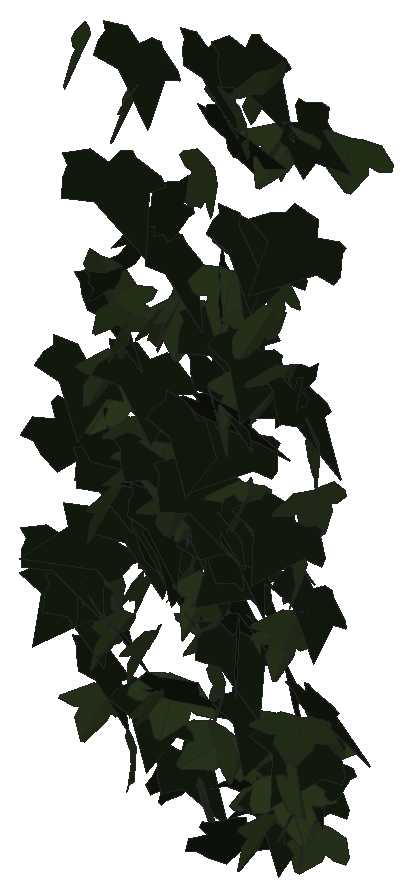
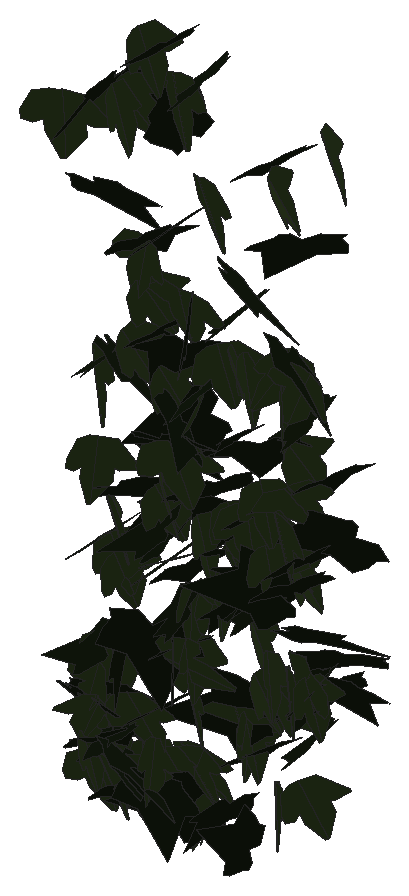
# SketchUp Ruby script. Lengths in inches.
U = 1.inch
M = Sketchup.active_model
def pt(a) = Geom::Point3d.new(a.map { |v| v * U })
def face(e, loops, mat)
  f = e.add_face(loops[0].map { |a| pt(a) })
  loops[1..].each { |l| e.add_face(l.map { |a| pt(a) }).erase! }
  f.material = f.back_material = mat if mat
  f
end
# faces: each face lists its corners as indices into pts; further lists are holes
def faces(e, pts, list, mat = nil) = list.each { |f| face(e, (f[0].is_a?(Array) ? f : [f]).map { |l| l.map { |i| pts[i] } }, mat) }
# xy, xz, yz: faces in a plane at the given z, y or x. An outline is a flat list of corners, or four numbers for a rectangle; further outlines are holes
def ring(l) = l.size == 4 ? [[l[0], l[1]], [l[2], l[1]], [l[2], l[3]], [l[0], l[3]]] : l.each_slice(2).to_a
def flat(e, list, mat, &to3) = list.each { |f| face(e, (f[0].is_a?(Array) ? f : [f]).map { |l| ring(l).map { |u, v| to3.(u, v) } }, mat) }
def xy(e, z, list, mat = nil) = flat(e, list, mat) { |x, y| [x, y, z] }
def xz(e, y, list, mat = nil) = flat(e, list, mat) { |x, z| [x, y, z] }
def yz(e, x, list, mat = nil) = flat(e, list, mat) { |y, z| [x, y, z] }
def lines(e, pts, list) = list.each { |a, b| e.add_line(pt(pts[a]), pt(pts[b])) }
# prism: a flat outline (further loops are holes) pulled along v
def prism(e, loops, v, mat = nil)
  f = face(e, loops, mat); d = Geom::Vector3d.new(v.map { |x| x * U })
  f.pushpull(f.normal.samedirection?(d) ? d.length : -d.length)
end
def box(e, o, s, mat = nil) = prism(e, [[o, [o[0] + s[0], o[1], o[2]], [o[0] + s[0], o[1] + s[1], o[2]], [o[0], o[1] + s[1], o[2]]]], [0, 0, s[2]], mat)
def at(x, y, z, deg = 0) = Geom::Transformation.translation(pt([x, y, z])) * Geom::Transformation.rotation(ORIGIN, Z_AXIS, deg.degrees)
def axes(o, x, y, z) = Geom::Transformation.new([*x, 0, *y, 0, *z, 0, *pt(o).to_a, 1])
def part(name) = M.definitions.add(name)
# library, detail: a bought-in or finely detailed component or shape, given as its bounding box
def library(name, o, s) = part(name).tap { |d| box(d.entities, o, s) }
def detail(e, o, s) = box(e.add_group.entities, o, s)
def put(e, d, t, mat = nil) = e.add_instance(d, t).tap { |i| i.material = mat if mat }
def group(e, t, mat = nil) = e.add_group.tap { |g| g.transformation = t; g.material = mat if mat }.entities
root = M.entities
M.materials.add("1026 AP 7946 SUNNY SIDE UP").color = [254, 231, 186]
M.materials.add("efeu1").color = [18, 25, 13]
M.materials.add("efeu2").color = [43, 57, 29]
c1 = part("ivyleaf_9")
p = [[1.54,2.16,1.25],[1.36,2.04,1.19],[-0.21,0.99,0.68],[-0.71,1.11,0.82],[-0.85,0.86,0.67],[-0.8,0.17,0.21],
  [-0.9,-0.01,0.1],[-0.67,-0.16,-0.02],[-0.08,-0.08,-0.05],[-0.03,-0.6,-0.4],[0.65,-0.88,-0.66],[0.83,-0.6,-0.49],
  [1.29,-0.42,-0.43],[1.8125,-0.07,-0.26],[1.21,0.44,0.15]]
faces(c1.entities,p,[[0,1,2,3,4,5,6,7,8,9,10,11,12,13,14]],"efeu1")
c2 = part("ivyleaf_10")
p = [[0,0.5,-0.03],[-0.0625,2.02,-0.43],[-0.19,2.01,-0.46],[-0.54,1.05,-0.29],[-0.52,0.625,-0.18],[-0.83,0.76,-0.28],
  [-1.16,0.64,-0.33],[-1.15,0.33,-0.24],[-0.77,-0.39,0.02],[-0.3,-0.51,0.16],[0.04,-0.48,0.23],[-0.02,2.01,-0.4375],
  [-0.06,2.01,-0.43],[0.04,-0.49,0.23],[0.67,-0.49,0.14],[1.38,0.36,-0.2],[1.375,0.51,-0.24],[0.81,0.65,-0.19],
  [0.62,0.59,-0.15],[0.6,1.09,-0.28],[0.5,1.23,-0.31]]
faces(c2.entities,p,[[0,1,2,3,4,5,6,7,8,9,10],[11,12,0,13,14,15,16,17,18,19,20]],"efeu2")
put(root,c1,axes([121.98,212.34,282.11],[-0.4716,-0.12043,-0.03746],[0.06512,-0.00764,-0.3322],[0.18645,-0.30194,0.02129]),"1026 AP 7946 SUNNY SIDE UP")
put(root,c2,axes([122.47,212.32,283.62],[0.07982,-0.31005,0.11549],[0.01592,-0.11369,-0.32422],[0.51911,0.05116,-0.00781]),"1026 AP 7946 SUNNY SIDE UP")
put(root,c1,axes([124.34,212.375,289.46],[0.07337,-0.12102,0.34642],[0.30772,-0.27593,-0.13163],[0.47142,0.19895,0.03201]),"1026 AP 7946 SUNNY SIDE UP")
put(root,c2,axes([125.5,212.28,282.88],[-0.20224,-0.29102,0.07419],[-0.01458,-0.07625,-0.32746],[0.47181,-0.1271,0.02168]),"1026 AP 7946 SUNNY SIDE UP")
put(root,c2,axes([125.39,212.33,282.65],[-0.14641,-0.29461,0.11515],[0.04803,-0.12613,-0.31235],[0.49408,-0.07504,0.06448]),"1026 AP 7946 SUNNY SIDE UP")
put(root,c2,axes([123.88,212.42,282.69],[-0.06359,-0.22295,0.24256],[0.12672,-0.23798,-0.2181],[0.49536,0.03226,0.08693]),"1026 AP 7946 SUNNY SIDE UP")
put(root,c2,axes([125.38,212.2,280.39],[0.3979,0.18623,0.0915],[0.1379,0.0283,-0.32221],[-0.29287,0.26634,-0.02741]),"1026 AP 7946 SUNNY SIDE UP")
put(root,c1,axes([122.46,212.29,288.4375],[-0.09486,-0.31906,-0.17967],[0.11042,0.16139,-0.33169],[0.55961,-0.08593,0.03499]),"1026 AP 7946 SUNNY SIDE UP")
put(root,c1,axes([124.34,212.03,279.43],[0.08612,0.14579,-0.28237],[0.14093,0.25993,0.16191],[0.46857,-0.10497,0.0032]),"1026 AP 7946 SUNNY SIDE UP")
put(root,c2,axes([125.61,212.26,281.38],[-0.3918,-0.209,0.04614],[-0.03482,-0.045,-0.33466],[0.33468,-0.24935,0.01919]),"1026 AP 7946 SUNNY SIDE UP")
put(root,c1,axes([123.72,212.48,285.05],[-0.12021,-0.32303,0.09626],[-0.00443,-0.09708,-0.34199],[0.52955,-0.07414,0.01899]),"1026 AP 7946 SUNNY SIDE UP")
put(root,c2,axes([124.93,212.41,279.61],[0.00787,-0.27161,0.17281],[0.01371,-0.16913,-0.2808],[0.50306,0.00886,0.00495]),"1026 AP 7946 SUNNY SIDE UP")
put(root,c2,axes([122.54,212.43,281.72],[0.00962,-0.26489,0.19993],[0.01872,-0.19531,-0.27404],[0.51741,0.01199,0.0062]),"1026 AP 7946 SUNNY SIDE UP")
put(root,c1,axes([123.28,212.51,282.92],[0.00139,-0.22449,0.25658],[0.02304,-0.25007,-0.23254],[0.52821,0.0115,0.00947]),"1026 AP 7946 SUNNY SIDE UP")
put(root,c1,axes([123.11,212.47,280.73],[-0.15088,-0.29808,0.07784],[0.0184,-0.08438,-0.32097],[0.48384,-0.08974,0.03648]),"1026 AP 7946 SUNNY SIDE UP")
put(root,c1,axes([122.2,212.38,281.18],[0.14885,-0.30447,0.0188],[-0.0019,-0.0213,-0.32851],[0.47977,0.09438,-0.00714]),"1026 AP 7946 SUNNY SIDE UP")
put(root,c2,axes([122.9,212.19,280.05],[0.20398,-0.25965,-0.14636],[0.00861,0.15566,-0.29003],[0.46421,0.11121,0.06969]),"1026 AP 7946 SUNNY SIDE UP")
put(root,c2,axes([123.58,212.3,283.99],[-0.16181,-0.31981,0.00986],[-0.00055,-0.01185,-0.34616],[0.5032,-0.10285,0.00279]),"1026 AP 7946 SUNNY SIDE UP")
put(root,c1,axes([124.7,212.51,286.4],[-0.13871,-0.31108,0.10614],[-0.01949,-0.10528,-0.33332],[0.51579,-0.08763,0.01595]),"1026 AP 7946 SUNNY SIDE UP")
put(root,c1,axes([121.9375,212.35,282.08],[-0.0157,-0.30585,-0.11025],[-0.00953,0.10549,-0.3145],[0.50853,-0.00747,-0.0093]),"1026 AP 7946 SUNNY SIDE UP")
put(root,c1,axes([123.85,212.34,284.39],[0.043,-0.35183,-0.15438],[0.05737,0.14997,-0.3598],[0.59734,0.01092,0.04567]),"1026 AP 7946 SUNNY SIDE UP")
put(root,c2,axes([123.45,212.33,281.13],[0.4817,0.10245,-0.03466],[-0.03828,-0.03479,-0.33198],[-0.16548,0.30629,-0.0241]),"1026 AP 7946 SUNNY SIDE UP")
put(root,c2,axes([123.03,212.37,281.71],[0.02886,-0.31487,0.06319],[-0.00167,-0.06329,-0.32526],[0.50495,0.01779,-0.00469]),"1026 AP 7946 SUNNY SIDE UP")
put(root,c1,axes([123.11,212.48,283.58],[0.06851,-0.32896,0.07609],[0.00669,-0.07582,-0.34225],[0.53074,0.04342,-0.00551]),"1026 AP 7946 SUNNY SIDE UP")
put(root,c1,axes([121.66,212.39,282.65],[-0.10323,-0.28278,-0.15401],[0.23333,0.10662,-0.27726],[0.44423,-0.12171,0.10984]),"1026 AP 7946 SUNNY SIDE UP")
put(root,c1,axes([124.45,212.57,283.15],[-0.31501,-0.19963,0.17381],[-0.04205,-0.1971,-0.2723],[0.40999,-0.1736,0.10562]),"1026 AP 7946 SUNNY SIDE UP")
put(root,c2,axes([125.3125,212.46,289.74],[-0.28616,-0.237,0.19736],[-0.06715,-0.20262,-0.29911],[0.4758,-0.17113,0.07648]),"1026 AP 7946 SUNNY SIDE UP")
put(root,c1,axes([123.33,212.2,281.125],[0.40036,-0.00071,0.20678],[0.31555,0.00781,-0.26217],[-0.00673,0.32413,0.00866]),"1026 AP 7946 SUNNY SIDE UP")
put(root,c2,axes([121.95,212.35,290.03],[0.21551,-0.3307,-0.02537],[-0.01643,0.02029,-0.36866],[0.52096,0.13744,-0.00113]),"1026 AP 7946 SUNNY SIDE UP")
put(root,c1,axes([124.46,212.53,283.46],[0.10075,-0.28666,0.17582],[0.04375,-0.17025,-0.30347],[0.52407,0.06932,-0.00847]),"1026 AP 7946 SUNNY SIDE UP")
put(root,c2,axes([125.64,212.14,280.33],[-0.04654,0.27766,-0.20714],[-0.0628,0.19924,0.28841],[0.53684,0.04738,0.01578]),"1026 AP 7946 SUNNY SIDE UP")
put(root,c2,axes([123.24,212.35,280.96],[-0.02999,-0.31993,-0.01573],[0.01456,0.01292,-0.32998],[0.50329,-0.01944,0.00861]),"1026 AP 7946 SUNNY SIDE UP")
put(root,c1,axes([121.87,212.54,285.23],[-0.13038,-0.32634,0.05369],[-0.00101,-0.05548,-0.34695],[0.52011,-0.08192,0.01279]),"1026 AP 7946 SUNNY SIDE UP")
put(root,c1,axes([123.03,212.47,282.96],[0.24152,-0.28204,0.07856],[0.03383,-0.07681,-0.33082],[0.45882,0.15413,-0.01696]),"1026 AP 7946 SUNNY SIDE UP")
put(root,c2,axes([124.9375,212.4,290.56],[-0.0761,-0.35302,0.02445],[0.0011,-0.02608,-0.36721],[0.55657,-0.04822,0.00407]),"1026 AP 7946 SUNNY SIDE UP")
put(root,c1,axes([124.31,212.3,283.96],[0.04677,-0.22517,-0.25324],[0.1103,0.24424,-0.22147],[0.51093,-0.03211,0.07099]),"1026 AP 7946 SUNNY SIDE UP")
put(root,c1,axes([122.97,212.48,283.41],[-0.25344,-0.25116,-0.14727],[0.24254,0.06186,-0.29369],[0.38297,-0.20538,0.08854]),"1026 AP 7946 SUNNY SIDE UP")
put(root,c2,axes([124.81,212.5,286.96],[-0.1432,-0.28736,0.16861],[-0.01065,-0.16978,-0.30889],[0.52116,-0.08242,0.04002]),"1026 AP 7946 SUNNY SIDE UP")
put(root,c2,axes([125.47,212.3,280.1],[0.10436,-0.29396,-0.11603],[-0.00971,0.11216,-0.30927],[0.49395,0.06431,0.01844]),"1026 AP 7946 SUNNY SIDE UP")
put(root,c1,axes([122.35,212.52,282.8],[-0.46019,-0.02794,0.14917],[-0.20323,-0.10704,-0.2907],[0.11217,-0.30856,0.08531]),"1026 AP 7946 SUNNY SIDE UP")
put(root,c2,axes([122.3,212.53,285.41],[-0.05315,-0.2918,0.17885],[0.02478,-0.17728,-0.30197],[0.53466,-0.0208,0.03177]),"1026 AP 7946 SUNNY SIDE UP")
put(root,c2,axes([124.49,212.26,289.96],[0.39965,-0.1725,-0.1954],[-0.10129,0.21428,-0.28995],[0.38903,0.23301,0.12524]),"1026 AP 7946 SUNNY SIDE UP")
put(root,c1,axes([125.18,212.62,284.02],[-0.30683,-0.25694,0.08238],[-0.02483,-0.08945,-0.33031],[0.42309,-0.19159,0.04036]),"1026 AP 7946 SUNNY SIDE UP")
put(root,c2,axes([123.28,212.3125,281.01],[-0.01538,-0.29711,-0.15278],[0.02307,0.14614,-0.30525],[0.52045,-0.01526,0.00901]),"1026 AP 7946 SUNNY SIDE UP")
put(root,c2,axes([122.68,212.26,286.51],[-0.20494,-0.22646,-0.23116],[0.20839,0.18046,-0.26741],[0.45434,-0.18492,0.01838]),"1026 AP 7946 SUNNY SIDE UP")
put(root,c1,axes([124.45,212.64,288],[-0.0305,-0.33944,0.09793],[-0.00525,-0.09695,-0.35082],[0.55508,-0.01957,0.00206]),"1026 AP 7946 SUNNY SIDE UP")
put(root,c1,axes([122.08,212.49,281.94],[0.33523,-0.2461,0.01976],[-0.00104,-0.02775,-0.33505],[0.38832,0.21238,-0.01795]),"1026 AP 7946 SUNNY SIDE UP")
put(root,c2,axes([122.2,212.53,280.49],[-0.22903,-0.26725,0.12402],[-0.02738,-0.12797,-0.31121],[0.46107,-0.14036,0.04312]),"1026 AP 7946 SUNNY SIDE UP")
put(root,c1,axes([121.6,212.34,284.39],[0.131,-0.10674,-0.32984],[0.3227,0.27715,-0.03863],[0.42016,-0.17959,0.13251]),"1026 AP 7946 SUNNY SIDE UP")
put(root,c1,axes([125.53,212.58,280.92],[-0.42097,-0.16263,-0.03561],[0.0694,-0.00816,-0.3213],[0.25174,-0.26971,0.02904]),"1026 AP 7946 SUNNY SIDE UP")
put(root,c2,axes([125.02,212.5625,286.16],[-0.0173,-0.32197,0.13866],[-0.01208,-0.13624,-0.33267],[0.54971,-0.01313,-0.00295]),"1026 AP 7946 SUNNY SIDE UP")
put(root,c2,axes([125.46,212.4,283.53],[0.22409,-0.28692,-0.11677],[-0.07305,0.10166,-0.32942],[0.4786,0.14985,0.0044]),"1026 AP 7946 SUNNY SIDE UP")
put(root,c1,axes([125.49,212.65,283.14],[-0.04575,-0.31576,0.10912],[0.01345,-0.1088,-0.32681],[0.52442,-0.02476,0.0179]),"1026 AP 7946 SUNNY SIDE UP")
put(root,c2,axes([124.42,212.59,285.85],[-0.08887,-0.29048,0.16641],[0.05685,-0.16988,-0.29963],[0.52079,-0.03102,0.0611]),"1026 AP 7946 SUNNY SIDE UP")
put(root,c1,axes([125.55,212.6,288.32],[-0.52722,-0.08548,-0.01484],[0.03195,-0.02355,-0.35545],[0.13238,-0.33476,0.0267]),"1026 AP 7946 SUNNY SIDE UP")
put(root,c2,axes([124.07,212.4375,285.53],[-0.17064,0.31483,-0.05166],[0.01132,-0.05243,-0.34321],[-0.5016,-0.10829,0.00983]),"1026 AP 7946 SUNNY SIDE UP")
put(root,c2,axes([124.54,212.46,284.23],[0.13973,-0.32884,-0.05482],[-0.01609,0.05042,-0.35061],[0.52309,0.08939,0.00386]),"1026 AP 7946 SUNNY SIDE UP")
put(root,c2,axes([123.6875,212.36,282.96],[0.02475,-0.27978,-0.17698],[-0.01887,0.16979,-0.28768],[0.51459,0.01968,-0.00204]),"1026 AP 7946 SUNNY SIDE UP")
put(root,c1,axes([123.82,212.62,290.45],[0.13275,-0.34153,0.05339],[0.00534,-0.05452,-0.36261],[0.54361,0.08394,-0.00948]),"1026 AP 7946 SUNNY SIDE UP")
put(root,c2,axes([125.78,212.3,285.5],[0.28543,-0.23687,-0.25889],[-0.08452,0.25961,-0.29214],[0.53485,0.16744,0.09199]),"1026 AP 7946 SUNNY SIDE UP")
put(root,c1,axes([124.52,212.53,290.73],[0.12866,-0.33682,-0.11172],[0.00366,0.10986,-0.35535],[0.55546,0.07729,0.02822]),"1026 AP 7946 SUNNY SIDE UP")
put(root,c2,axes([125.67,212.52,279.72],[-0.4649,-0.02703,0.10382],[-0.13619,-0.10602,-0.29126],[0.0919,-0.29388,0.09356]),"1026 AP 7946 SUNNY SIDE UP")
put(root,c1,axes([122.22,212.55,283.94],[0.05745,-0.31882,-0.09316],[0.00423,0.08944,-0.32983],[0.5203,0.03448,0.01297]),"1026 AP 7946 SUNNY SIDE UP")
put(root,c2,axes([123.23,212.56,283.48],[0.43217,-0.18044,0.03736],[0.02743,-0.04119,-0.33799],[0.28842,0.27429,-0.02384]),"1026 AP 7946 SUNNY SIDE UP")
put(root,c1,axes([125.29,212.5625,285.99],[0.19565,-0.32,-0.05768],[-0.01703,0.05389,-0.35326],[0.51005,0.12455,0.01033]),"1026 AP 7946 SUNNY SIDE UP")
put(root,c1,axes([124.75,212.72,287.86],[-0.23055,-0.30394,0.07165],[-0.0215,-0.07242,-0.34754],[0.49041,-0.14606,0.01845]),"1026 AP 7946 SUNNY SIDE UP")
put(root,c2,axes([122.94,212.55,282.58],[0.12885,-0.32576,0.01274],[-0.00139,-0.01488,-0.34611],[0.51271,0.08183,-0.00414]),"1026 AP 7946 SUNNY SIDE UP")
put(root,c1,axes([123.93,212.4,285.42],[0.51764,-0.0153,0.07172],[0.10966,-0.00084,-0.33951],[0.02382,0.3365,0.00438]),"1026 AP 7946 SUNNY SIDE UP")
put(root,c1,axes([124.56,212.73,280.97],[-0.13617,-0.28603,0.12355],[-0.00739,-0.12496,-0.30712],[0.48863,-0.0816,0.02979]),"1026 AP 7946 SUNNY SIDE UP")
put(root,c2,axes([123.85,212.49,279.61],[-0.23947,0.27075,-0.03908],[0.02113,-0.03772,-0.32016],[-0.4297,-0.15274,0.00604]),"1026 AP 7946 SUNNY SIDE UP")
put(root,c1,axes([122.89,212.53,284.42],[0.12134,-0.295,-0.15184],[-0.00696,0.14873,-0.31173],[0.51732,0.07119,0.03142]),"1026 AP 7946 SUNNY SIDE UP")
put(root,c2,axes([122.59,212.46,286.1],[0.10826,-0.31779,-0.12598],[0.0261,0.12593,-0.33168],[0.53377,0.0583,0.04177]),"1026 AP 7946 SUNNY SIDE UP")
put(root,c2,axes([124.11,212.45,281.32],[0.23118,-0.26541,-0.15072],[-0.06006,0.14342,-0.30993],[0.47159,0.14837,0.03442]),"1026 AP 7946 SUNNY SIDE UP")
put(root,c2,axes([123.87,212.47,288.74],[0.35539,-0.22568,-0.15131],[-0.10772,0.13555,-0.32523],[0.40833,0.23218,0.0459]),"1026 AP 7946 SUNNY SIDE UP")
put(root,c2,axes([125.21,212.64,279.79],[0.27751,-0.18782,0.17857],[0.24236,-0.09141,-0.26263],[0.322,0.23067,0.04378]),"1026 AP 7946 SUNNY SIDE UP")
put(root,c1,axes([124.21,212.55,283.36],[0.20725,-0.29559,-0.10889],[-0.02023,0.10765,-0.3313],[0.49232,0.12886,0.03223]),"1026 AP 7946 SUNNY SIDE UP")
put(root,c2,axes([123.88,212.53,283.78],[0.02193,-0.33717,-0.04413],[0.00047,0.04097,-0.3474],[0.53405,0.01381,0.00212]),"1026 AP 7946 SUNNY SIDE UP")
put(root,c1,axes([124.39,212.7,285],[-0.4866,-0.13385,-0.00032],[0.01683,-0.02587,-0.3463],[0.20979,-0.30838,0.02703]),"1026 AP 7946 SUNNY SIDE UP")
put(root,c1,axes([123.99,212.72,283.33],[-0.10047,-0.32563,0.01998],[-0.00684,-0.0208,-0.34199],[0.51307,-0.06404,-0.00065]),"1026 AP 7946 SUNNY SIDE UP")
put(root,c1,axes([124.19,212.66,281.97],[-0.00722,-0.32103,-0.06229],[0.04487,0.05803,-0.32922],[0.51118,-0.00963,0.02802]),"1026 AP 7946 SUNNY SIDE UP")
put(root,c2,axes([122.84,212.58,284.6875],[-0.20818,-0.30536,0.00871],[0.00493,-0.01247,-0.34285],[0.48039,-0.1322,0.00729]),"1026 AP 7946 SUNNY SIDE UP")
put(root,c1,axes([125.42,212.77,280.3],[-0.26727,-0.26396,0.05996],[0.00758,-0.07345,-0.32081],[0.42547,-0.1645,0.04338]),"1026 AP 7946 SUNNY SIDE UP")
put(root,c1,axes([121.96,212.62,282.17],[0.21505,-0.2968,-0.07084],[-0.06752,0.05398,-0.33594],[0.47368,0.14244,-0.01573]),"1026 AP 7946 SUNNY SIDE UP")
put(root,c2,axes([124.41,212.69,284.14],[-0.17738,-0.28406,0.14147],[0.0116,-0.14984,-0.3103],[0.49709,-0.09787,0.05772]),"1026 AP 7946 SUNNY SIDE UP")
put(root,c1,axes([122.78,212.71,285.5],[-0.22172,-0.30065,-0.08306],[0.07222,0.06556,-0.34144],[0.4834,-0.14769,0.01291]),"1026 AP 7946 SUNNY SIDE UP")
put(root,c2,axes([123.47,212.66,286.52],[-0.28908,-0.28375,0.07992],[0.01793,-0.10013,-0.34293],[0.46287,-0.17333,0.0632]),"1026 AP 7946 SUNNY SIDE UP")
put(root,c1,axes([123.12,212.71,287.33],[0.13543,-0.33564,0.00253],[-0.00632,-0.00554,-0.35697],[0.52777,0.08606,-0.00493]),"1026 AP 7946 SUNNY SIDE UP")
put(root,c1,axes([125.84,212.65,280.75],[-0.48537,0.07043,0.01745],[-0.03725,-0.02992,-0.32442],[-0.10748,-0.30767,0.03363]),"1026 AP 7946 SUNNY SIDE UP")
put(root,c2,axes([124.01,212.55,282.74],[-0.04931,-0.32496,-0.0914],[0.06386,0.08295,-0.33429],[0.52505,-0.04061,0.03208]),"1026 AP 7946 SUNNY SIDE UP")
put(root,c2,axes([124.11,212.625,287.15],[0.52669,-0.05881,0.01641],[0.02566,-0.00111,-0.35035],[0.09245,0.33535,0.00374]),"1026 AP 7946 SUNNY SIDE UP")
put(root,c1,axes([123.84,212.6875,285.83],[0.1722,-0.32181,-0.00948],[0.00243,0.00831,-0.35012],[0.50614,0.10945,0.0049]),"1026 AP 7946 SUNNY SIDE UP")
put(root,c2,axes([122.51,212.71,289.36],[0.1922,-0.30803,0.10394],[0.03418,-0.10166,-0.34157],[0.50939,0.12305,-0.0163]),"1026 AP 7946 SUNNY SIDE UP")
put(root,c2,axes([124.02,212.61,280.43],[0.40839,-0.04233,-0.17311],[-0.26307,0.01594,-0.27083],[0.06956,0.3088,-0.00791]),"1026 AP 7946 SUNNY SIDE UP")
put(root,c1,axes([124.45,212.4,282.03],[0.06776,-0.02168,-0.33577],[-0.43625,0.17087,-0.04852],[0.27075,0.28074,0.00586]),"1026 AP 7946 SUNNY SIDE UP")
put(root,c2,axes([125.2,212.62,289.71],[0.02136,-0.35604,-0.00922],[0.01067,0.00719,-0.36695],[0.55985,0.01345,0.00735]),"1026 AP 7946 SUNNY SIDE UP")
put(root,c2,axes([123.23,212.66,286.52],[0.19477,-0.32447,0.01506],[0.00449,-0.01653,-0.35788],[0.51083,0.12386,-0.0026]),"1026 AP 7946 SUNNY SIDE UP")
put(root,c1,axes([123.17,212.67,283.04],[0.02392,-0.30699,-0.10376],[0.01166,0.09939,-0.31583],[0.50704,0.0122,0.01216]),"1026 AP 7946 SUNNY SIDE UP")
put(root,c2,axes([123.05,212.64,284.31],[-0.35594,-0.24561,0.03438],[0.0164,-0.05645,-0.3412],[0.3897,-0.22196,0.04576]),"1026 AP 7946 SUNNY SIDE UP")
put(root,c1,axes([124.97,212.79,279.78],[-0.15219,-0.30122,0.03255],[0.00916,-0.03681,-0.32571],[0.47644,-0.09551,0.01666]),"1026 AP 7946 SUNNY SIDE UP")
put(root,c2,axes([124.86,212.58,287.59],[-0.45861,0.18111,0.00674],[-0.04852,-0.03935,-0.35019],[-0.28074,-0.28905,0.04951]),"1026 AP 7946 SUNNY SIDE UP")
put(root,c2,axes([122.01,212.67,282.28],[0.3629,-0.16423,0.17168],[0.28642,-0.02276,-0.28155],[0.23256,0.28431,0.07886]),"1026 AP 7946 SUNNY SIDE UP")
put(root,c2,axes([123.11,212.57,286.45],[0.0174,-0.33746,-0.09425],[-0.00988,0.08941,-0.34729],[0.5489,0.01231,-0.00326]),"1026 AP 7946 SUNNY SIDE UP")
put(root,c1,axes([125.42,212.67,281.58],[0.28607,-0.25561,0.03161],[0.08715,0.00042,-0.31985],[0.39559,0.18475,0.0476]),"1026 AP 7946 SUNNY SIDE UP")
put(root,c2,axes([124.05,212.56,280.43],[0.34869,-0.13398,-0.17911],[-0.20083,0.12091,-0.26427],[0.27953,0.25401,0.03356]),"1026 AP 7946 SUNNY SIDE UP")
put(root,c2,axes([122.5,212.64,284.39],[0.38482,-0.23632,-0.02074],[0.02684,0.0445,-0.3473],[0.3718,0.24138,0.04654]),"1026 AP 7946 SUNNY SIDE UP")
put(root,c2,axes([124.94,212.65,280.87],[-0.42564,0.00658,0.16081],[-0.23798,-0.08827,-0.26713],[0.06074,-0.29973,0.08029]),"1026 AP 7946 SUNNY SIDE UP")
put(root,c2,axes([122.27,212.73,284.96],[0.35527,0.19536,-0.16473],[-0.16816,-0.12195,-0.30775],[-0.3608,0.2492,-0.01877]),"1026 AP 7946 SUNNY SIDE UP")
put(root,c2,axes([122.4,212.57,282.08],[0.2234,-0.26924,-0.14321],[-0.00765,0.14985,-0.30663],[0.4753,0.12896,0.06238]),"1026 AP 7946 SUNNY SIDE UP")
put(root,c1,axes([124.02,212.69,286.53],[-0.1308,-0.27199,-0.20422],[0.1516,0.17474,-0.28992],[0.50555,-0.12277,0.0341]),"1026 AP 7946 SUNNY SIDE UP")
put(root,c2,axes([121.99,212.6875,282.14],[-0.08275,-0.31424,0.01373],[0.00569,-0.01592,-0.32826],[0.49464,-0.05239,0.00607]),"1026 AP 7946 SUNNY SIDE UP")
put(root,c1,axes([122.47,212.5,286.82],[-0.19302,0.30674,0.09065],[-0.059,0.07787,-0.33986],[-0.49755,-0.12823,0.00513]),"1026 AP 7946 SUNNY SIDE UP")
put(root,c2,axes([123.9,212.62,282.04],[-0.0635,-0.31388,-0.09083],[0.05635,0.08223,-0.32459],[0.50879,-0.04828,0.02461]),"1026 AP 7946 SUNNY SIDE UP")
put(root,c2,axes([124.92,212.67,279.99],[0.36013,-0.07747,-0.2086],[-0.31241,0.04127,-0.24808],[0.13481,0.30261,-0.01765]),"1026 AP 7946 SUNNY SIDE UP")
put(root,c1,axes([125.29,212.63,285.98],[-0.37033,0.24904,-0.02223],[-0.00602,-0.03517,-0.35223],[-0.39321,-0.23401,0.02633]),"1026 AP 7946 SUNNY SIDE UP")
put(root,c2,axes([122.63,212.72,283.86],[-0.15114,-0.32077,-0.00298],[0.01425,-0.0016,-0.34485],[0.50418,-0.09612,0.00885]),"1026 AP 7946 SUNNY SIDE UP")
put(root,c2,axes([122.11,212.7,286.64],[-0.46918,0.14429,-0.06778],[0.06113,-0.07113,-0.33853],[-0.24231,-0.29734,0.04584]),"1026 AP 7946 SUNNY SIDE UP")
put(root,c1,axes([123.35,212.68,279.98],[0.08743,-0.24784,-0.20207],[-0.05725,0.19137,-0.2605],[0.4923,0.06627,0.00559]),"1026 AP 7946 SUNNY SIDE UP")
put(root,c1,axes([121.875,212.8125,286.22],[0.22204,-0.30562,0.01156],[0.00659,-0.01234,-0.3469],[0.48094,0.14126,-0.00059]),"1026 AP 7946 SUNNY SIDE UP")
put(root,c2,axes([124.21,212.75,284.87],[-0.4754,-0.10322,0.10859],[-0.13079,-0.08084,-0.326],[0.19239,-0.31002,0.04671]),"1026 AP 7946 SUNNY SIDE UP")
put(root,c1,axes([125.1,212.91,280.4],[0.04843,-0.28931,0.1193],[0.07732,-0.11205,-0.29829],[0.48484,0.04677,0.03565]),"1026 AP 7946 SUNNY SIDE UP")
put(root,c1,axes([122.18,212.86,283.71],[-0.08443,-0.31769,-0.03936],[0.02937,0.03374,-0.33147],[0.50195,-0.05541,0.01277]),"1026 AP 7946 SUNNY SIDE UP")
put(root,c2,axes([125.59,212.75,280.16],[0.03382,-0.31858,-0.0269],[-0.00003,0.02436,-0.3288],[0.50239,0.02145,0.00179]),"1026 AP 7946 SUNNY SIDE UP")
put(root,c1,axes([123.98,212.77,282.71],[0.33018,-0.26124,-0.04821],[-0.06552,0.02457,-0.3447],[0.41173,0.21341,-0.01619]),"1026 AP 7946 SUNNY SIDE UP")
put(root,c1,axes([122.42,212.9375,289.9],[-0.05947,-0.34456,0.026],[0.03297,-0.02959,-0.35641],[0.54247,-0.03598,0.02451]),"1026 AP 7946 SUNNY SIDE UP")
put(root,c2,axes([125.47,212.71,284.48],[-0.2418,-0.28964,-0.08294],[0.06791,0.06634,-0.33737],[0.4671,-0.15958,0.00612]),"1026 AP 7946 SUNNY SIDE UP")
put(root,c2,axes([125.56,212.71,281.1875],[-0.38623,0.19973,0.01042],[-0.03255,-0.01126,-0.32544],[-0.31268,-0.24554,0.02101]),"1026 AP 7946 SUNNY SIDE UP")
put(root,c1,axes([125.34,212.61,289.92],[0.23472,-0.15639,-0.2873],[-0.18902,0.25671,-0.21378],[0.46455,0.18347,0.05817]),"1026 AP 7946 SUNNY SIDE UP")
put(root,c1,axes([123.17,212.83,287.89],[-0.44942,0.16962,-0.08915],[0.07887,-0.08528,-0.33957],[-0.28956,-0.28649,0.04589]),"1026 AP 7946 SUNNY SIDE UP")
put(root,c1,axes([124.99,212.85,280.12],[-0.3869,0.1593,-0.1098],[0.07892,-0.11529,-0.29507],[-0.29168,-0.2425,0.0658]),"1026 AP 7946 SUNNY SIDE UP")
put(root,c2,axes([124.83,212.65,280.21],[-0.26597,0.21093,0.1686],[-0.20734,0.10084,-0.27573],[-0.36369,-0.21175,0.03389]),"1026 AP 7946 SUNNY SIDE UP")
put(root,c1,axes([125.1875,212.58,281.65],[0.12362,0.05035,-0.31173],[-0.43555,0.14651,-0.04812],[0.20827,0.2765,0.08439]),"1026 AP 7946 SUNNY SIDE UP")
put(root,c2,axes([125.45,212.75,280.79],[0.21256,0.28074,0.05021],[0.04194,0.03947,-0.32069],[-0.44564,0.13762,-0.00623]),"1026 AP 7946 SUNNY SIDE UP")
put(root,c2,axes([122.59,212.74,282.32],[0.03921,-0.29378,-0.16729],[-0.02744,0.15981,-0.30279],[0.52584,0.03024,-0.00333]),"1026 AP 7946 SUNNY SIDE UP")
put(root,c2,axes([125.22,212.82,279.96],[0.3032,-0.23,-0.09629],[-0.09586,0.06915,-0.30878],[0.37762,0.20222,-0.00108]),"1026 AP 7946 SUNNY SIDE UP")
put(root,c1,axes([123.07,212.64,279.42],[0.01345,-0.01278,0.3169],[0.31031,0.23652,0.00585],[-0.37173,0.19698,0.01635]),"1026 AP 7946 SUNNY SIDE UP")
put(root,c2,axes([124.46,212.77,280.41],[-0.0553,-0.30417,-0.14673],[0.05965,0.13695,-0.31397],[0.52358,-0.04773,0.02027]),"1026 AP 7946 SUNNY SIDE UP")
put(root,c1,axes([124.3,212.87,283.8],[0.33828,-0.24823,-0.02872],[0.02555,0.04879,-0.33505],[0.39169,0.21119,0.04666]),"1026 AP 7946 SUNNY SIDE UP")
put(root,c2,axes([124.18,212.83,281.93],[0.08739,-0.03971,-0.34005],[-0.50548,0.07804,-0.06502],[0.13194,0.32528,-0.02388]),"1026 AP 7946 SUNNY SIDE UP")
put(root,c1,axes([124.48,212.81,282.24],[0.29635,0.22084,-0.1765],[-0.14192,-0.14908,-0.29893],[-0.41723,0.20756,-0.02369]),"1026 AP 7946 SUNNY SIDE UP")
put(root,c1,axes([124.96,212.78,280.19],[-0.16879,0.27967,0.09349],[-0.14917,0.05679,-0.30084],[-0.4368,-0.12746,0.06661]),"1026 AP 7946 SUNNY SIDE UP")
put(root,c1,axes([124.125,212.67,285.35],[-0.00626,0.23484,0.25563],[0.01014,0.24683,-0.2404],[-0.53558,0.00193,-0.00754]),"1026 AP 7946 SUNNY SIDE UP")
put(root,c1,axes([123.96,212.7,287],[0.0522,0.07671,-0.34705],[-0.4519,0.19472,0.01762],[0.30274,0.27743,0.08614]),"1026 AP 7946 SUNNY SIDE UP")
put(root,c1,axes([124.37,212.83,279.95],[0.11853,0.2998,-0.026],[-0.07823,-0.01498,-0.31524],[-0.46679,0.07863,0.04623]),"1026 AP 7946 SUNNY SIDE UP")
put(root,c1,axes([122.47,212.79,283.46],[0.31266,0.0297,0.27195],[0.35258,0.15765,-0.19148],[-0.22346,0.29031,0.07838]),"1026 AP 7946 SUNNY SIDE UP")
put(root,c2,axes([125.82,213.01,289.59],[-0.50293,-0.12833,0.03241],[-0.02604,-0.04473,-0.35344],[0.2064,-0.31834,0.03439]),"1026 AP 7946 SUNNY SIDE UP")
